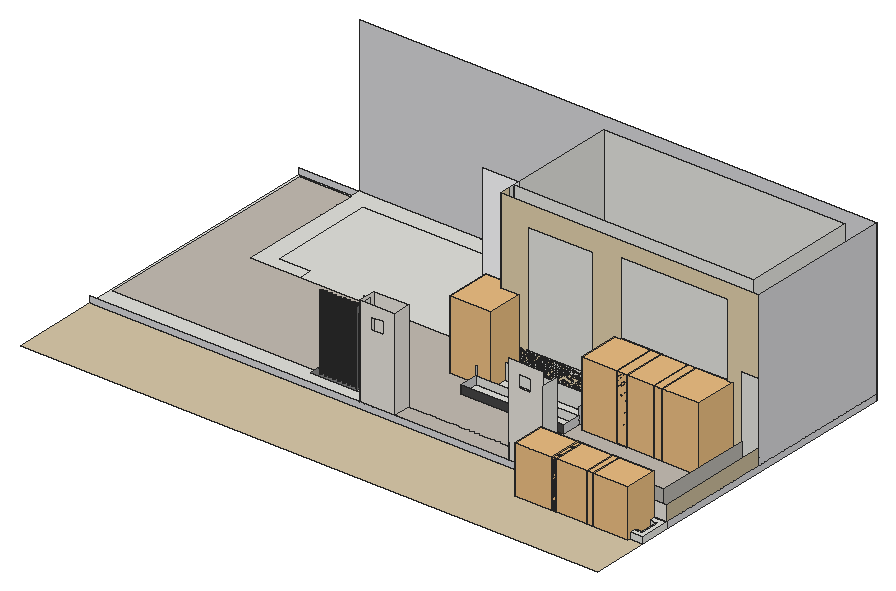
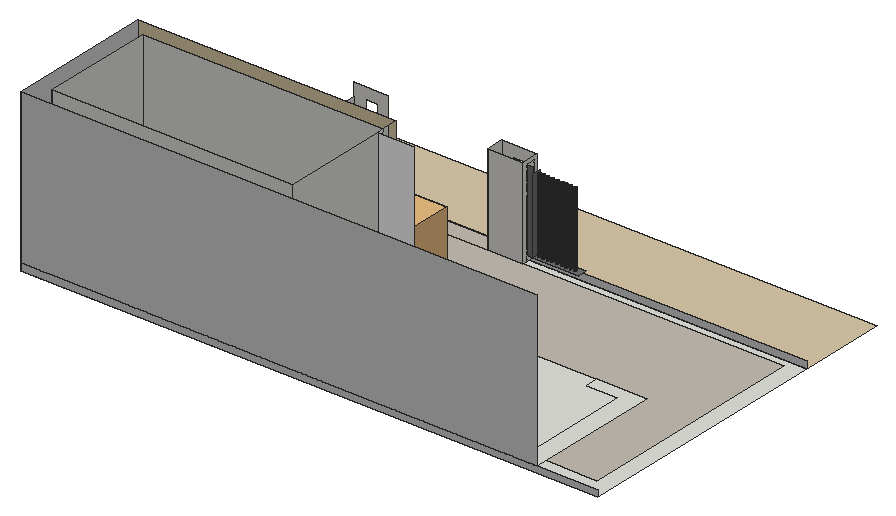
# SketchUp Ruby script. Lengths in inches.
U = 1.inch
M = Sketchup.active_model
def pt(a) = Geom::Point3d.new(a.map { |v| v * U })
def face(e, loops, mat)
  f = e.add_face(loops[0].map { |a| pt(a) })
  loops[1..].each { |l| e.add_face(l.map { |a| pt(a) }).erase! }
  f.material = f.back_material = mat if mat
  f
end
# faces: each face lists its corners as indices into pts; further lists are holes
def faces(e, pts, list, mat = nil) = list.each { |f| face(e, (f[0].is_a?(Array) ? f : [f]).map { |l| l.map { |i| pts[i] } }, mat) }
# xy, xz, yz: faces in a plane at the given z, y or x. An outline is a flat list of corners, or four numbers for a rectangle; further outlines are holes
def ring(l) = l.size == 4 ? [[l[0], l[1]], [l[2], l[1]], [l[2], l[3]], [l[0], l[3]]] : l.each_slice(2).to_a
def flat(e, list, mat, &to3) = list.each { |f| face(e, (f[0].is_a?(Array) ? f : [f]).map { |l| ring(l).map { |u, v| to3.(u, v) } }, mat) }
def xy(e, z, list, mat = nil) = flat(e, list, mat) { |x, y| [x, y, z] }
def xz(e, y, list, mat = nil) = flat(e, list, mat) { |x, z| [x, y, z] }
def yz(e, x, list, mat = nil) = flat(e, list, mat) { |y, z| [x, y, z] }
def lines(e, pts, list) = list.each { |a, b| e.add_line(pt(pts[a]), pt(pts[b])) }
# prism: a flat outline (further loops are holes) pulled along v
def prism(e, loops, v, mat = nil)
  f = face(e, loops, mat); d = Geom::Vector3d.new(v.map { |x| x * U })
  f.pushpull(f.normal.samedirection?(d) ? d.length : -d.length)
end
def box(e, o, s, mat = nil) = prism(e, [[o, [o[0] + s[0], o[1], o[2]], [o[0] + s[0], o[1] + s[1], o[2]], [o[0], o[1] + s[1], o[2]]]], [0, 0, s[2]], mat)
def at(x, y, z, deg = 0) = Geom::Transformation.translation(pt([x, y, z])) * Geom::Transformation.rotation(ORIGIN, Z_AXIS, deg.degrees)
def axes(o, x, y, z) = Geom::Transformation.new([*x, 0, *y, 0, *z, 0, *pt(o).to_a, 1])
def part(name) = M.definitions.add(name)
# library, detail: a bought-in or finely detailed component or shape, given as its bounding box
def library(name, o, s) = part(name).tap { |d| box(d.entities, o, s) }
def detail(e, o, s) = box(e.add_group.entities, o, s)
def put(e, d, t, mat = nil) = e.add_instance(d, t).tap { |i| i.material = mat if mat }
def group(e, t, mat = nil) = e.add_group.tap { |g| g.transformation = t; g.material = mat if mat }.entities
root = M.entities
M.materials.add("[Blinds Vertical Pattern]").color = [212, 212, 214]
M.materials.add("[Carrera Marble]").color = [207, 207, 207]
M.materials.add("[Color M05]").color = [114, 114, 114]
M.materials.add("[Field Rectangle Tile]").color = [196, 189, 179]
M.materials.add("[Field Square Tile]").color = [217, 201, 169]
M.materials.add("[Granite Dark Gray]").color = [69, 68, 68]
M.materials.add("[Quartz Light Brown]").color = [224, 207, 171]
M.materials.add("[Quartz Light Brown]1").color = [199, 184, 152]
M.materials.add("[Quartz Light Grey]").color = [251, 251, 252]
M.materials.add("[Tile Large Brown]").color = [195, 178, 159]
M.materials.add("[Tile Travertine 2 inch]").color = [229, 225, 218]
M.materials.add("[Tile Travertine 2 inch]1").color = [181, 178, 172]
c1 = library("chau cay",[-24.34,-109.24,0],[56.46,62.58,79.69])
c2 = library("Small+Bush+Planter",[-31.86,3.96,0],[62.63,58.8,106.375])
xy(root,0,[[[621.41,77.96,793.87,119.71],[628.97,85.52,786.3125,112.16]],[0,119.71,793.87,479.71]])
xy(root,0,[[0,0,0,119.71,621.41,119.71,621.41,77.96,793.87,77.96,793.87,0]],"[Field Square Tile]")
xy(root,0,[[628.97,85.52,786.3125,112.16]],"[Tile Large Brown]")
xy(root,8.625,[[[621.41,77.96,793.87,119.71],[628.97,85.52,786.3125,112.16]]])
xy(root,9,[[371.37,119.71,419.6875,143.63],[575.77,119.71,622.67,143.63],[622.67,119.71,622.67,143.63,769.95,143.63,769.95,277.72,793.87,277.72,793.87,119.71],[445.64,200.28,587.08,226.75],[445.64,226.75,587.08,253.22],
  [445.64,253.22,587.08,277.72],[769.95,277.72,769.95,455.8,107.23,455.8,107.23,309.84,151.04,309.84,151.04,291.34,83.3125,291.34,83.3125,479.71,793.87,479.71,793.87,277.72],[438.59,277.72,769.95,299.71],[388.47,291.34,438.59,299.71],[438.59,299.71,769.95,455.8]])
xy(root,9,[[419.6875,119.71,575.77,143.63],[12.5625,143.63,769.95,143.63,769.95,277.72,587.08,277.72,587.08,200.28,445.64,200.28,445.64,277.72,438.59,277.72,438.59,291.34,83.3125,291.34,83.3125,464.52,12.5625,464.52]],"[Field Rectangle Tile]")
xy(root,9,[[388.47,299.71,438.59,309.84]],"[Quartz Light Grey]")
xy(root,17.125,[[362.74,125.1875,371.37,137.375],[309.68,129.51,309.27,129.56,308.9,129.72,308.57,129.97,308.32,130.29,308.17,130.67,308.11,131.07,308.17,131.48,308.32,131.86,308.57,132.18,308.9,132.43,309.27,132.58,309.68,132.64,310.08,132.58,310.46,132.43,310.78,132.18,311.03,131.86,311.1875,131.48,311.24,131.07,311.1875,130.67,311.03,130.29,310.78,129.97,310.46,129.72,310.08,129.56],[315.49,129.51,315.09,129.56,314.71,129.72,314.38,129.97,314.14,130.29,313.98,130.67,313.93,131.07,313.98,131.48,314.14,131.86,314.38,132.18,314.71,132.43,315.09,132.58,315.49,132.64,315.89,132.58,316.27,132.43,316.59,132.18,316.84,131.86,317,131.48,317.05,131.07,317,130.67,316.84,130.29,316.59,129.97,316.27,129.72,315.89,129.56],[321.55,129.51,321.15,129.56,320.77,129.72,320.45,129.97,320.2,130.29,320.04,130.67,319.99,131.07,320.04,131.48,320.2,131.86,320.45,132.18,320.77,132.43,321.15,132.58,321.55,132.64,321.96,132.58,322.33,132.43,322.66,132.18,322.91,131.86,323.0625,131.48,323.11,131.07,323.0625,130.67,322.91,130.29,322.66,129.97,322.33,129.72,321.96,129.56],[327.61,129.51,327.21,129.56,326.83,129.72,326.51,129.97,326.26,130.29,326.11,130.67,326.05,131.07,326.11,131.48,326.26,131.86,326.51,132.18,326.83,132.43,327.21,132.58,327.61,132.64,328.02,132.58,328.4,132.43,328.72,132.18,328.97,131.86,329.125,131.48,329.18,131.07,329.125,130.67,328.97,130.29,328.72,129.97,328.4,129.72,328.02,129.56],
  [334.49,129.51,334.09,129.56,333.71,129.72,333.38,129.97,333.14,130.29,332.98,130.67,332.93,131.07,332.98,131.48,333.14,131.86,333.38,132.18,333.71,132.43,334.09,132.58,334.49,132.64,334.89,132.58,335.27,132.43,335.59,132.18,335.84,131.86,336,131.48,336.05,131.07,336,130.67,335.84,130.29,335.59,129.97,335.27,129.72,334.89,129.56],[340.86,129.51,340.46,129.56,340.08,129.72,339.76,129.97,339.51,130.29,339.36,130.67,339.3,131.07,339.36,131.48,339.51,131.86,339.76,132.18,340.08,132.43,340.46,132.58,340.86,132.64,341.27,132.58,341.65,132.43,341.97,132.18,342.22,131.86,342.375,131.48,342.43,131.07,342.375,130.67,342.22,130.29,341.97,129.97,341.65,129.72,341.27,129.56],[347.05,129.51,346.65,129.56,346.27,129.72,345.95,129.97,345.7,130.29,345.54,130.67,345.49,131.07,345.54,131.48,345.7,131.86,345.95,132.18,346.27,132.43,346.65,132.58,347.05,132.64,347.46,132.58,347.83,132.43,348.16,132.18,348.41,131.86,348.5625,131.48,348.61,131.07,348.5625,130.67,348.41,130.29,348.16,129.97,347.83,129.72,347.46,129.56],[353.05,129.51,352.65,129.56,352.27,129.72,351.95,129.97,351.7,130.29,351.54,130.67,351.49,131.07,351.54,131.48,351.7,131.86,351.95,132.18,352.27,132.43,352.65,132.58,353.05,132.64,353.46,132.58,353.83,132.43,354.16,132.18,354.41,131.86,354.5625,131.48,354.61,131.07,354.5625,130.67,354.41,130.29,354.16,129.97,353.83,129.72,353.46,129.56],[358.68,129.51,358.27,129.56,357.9,129.72,357.57,129.97,357.32,130.29,357.17,130.67,357.11,131.07,357.17,131.48,357.32,131.86,357.57,132.18,357.9,132.43,358.27,132.58,358.68,132.64,359.08,132.58,359.46,132.43,359.78,132.18,360.03,131.86,360.1875,131.48,360.24,131.07,360.1875,130.67,360.03,130.29,359.78,129.97,359.46,129.72,359.08,129.56]])
xy(root,17.125,[[[299.8,125.1875,362.74,137.375],[303.86,129.51,303.46,129.56,303.08,129.72,302.76,129.97,302.51,130.29,302.36,130.67,302.3,131.07,302.36,131.48,302.51,131.86,302.76,132.18,303.08,132.43,303.46,132.58,303.86,132.64,304.27,132.58,304.65,132.43,304.97,132.18,305.22,131.86,305.375,131.48,305.43,131.07,305.375,130.67,305.22,130.29,304.97,129.97,304.65,129.72,304.27,129.56],[358.68,129.51,358.27,129.56,357.9,129.72,357.57,129.97,357.32,130.29,357.17,130.67,357.11,131.07,357.17,131.48,357.32,131.86,357.57,132.18,357.9,132.43,358.27,132.58,358.68,132.64,359.08,132.58,359.46,132.43,359.78,132.18,360.03,131.86,360.1875,131.48,360.24,131.07,360.1875,130.67,360.03,130.29,359.78,129.97,359.46,129.72,359.08,129.56],[309.68,129.51,309.27,129.56,308.9,129.72,308.57,129.97,308.32,130.29,308.17,130.67,308.11,131.07,308.17,131.48,308.32,131.86,308.57,132.18,308.9,132.43,309.27,132.58,309.68,132.64,310.08,132.58,310.46,132.43,310.78,132.18,311.03,131.86,311.1875,131.48,311.24,131.07,311.1875,130.67,311.03,130.29,310.78,129.97,310.46,129.72,310.08,129.56],[353.05,129.51,352.65,129.56,352.27,129.72,351.95,129.97,351.7,130.29,351.54,130.67,351.49,131.07,351.54,131.48,351.7,131.86,351.95,132.18,352.27,132.43,352.65,132.58,353.05,132.64,353.46,132.58,353.83,132.43,354.16,132.18,354.41,131.86,354.5625,131.48,354.61,131.07,354.5625,130.67,354.41,130.29,354.16,129.97,353.83,129.72,353.46,129.56],[315.49,129.51,315.09,129.56,314.71,129.72,314.38,129.97,314.14,130.29,313.98,130.67,313.93,131.07,313.98,131.48,314.14,131.86,314.38,132.18,314.71,132.43,315.09,132.58,315.49,132.64,315.89,132.58,316.27,132.43,316.59,132.18,316.84,131.86,317,131.48,317.05,131.07,317,130.67,316.84,130.29,316.59,129.97,316.27,129.72,315.89,129.56],[347.05,129.51,346.65,129.56,346.27,129.72,345.95,129.97,345.7,130.29,345.54,130.67,345.49,131.07,345.54,131.48,345.7,131.86,345.95,132.18,346.27,132.43,346.65,132.58,347.05,132.64,347.46,132.58,347.83,132.43,348.16,132.18,348.41,131.86,348.5625,131.48,348.61,131.07,348.5625,130.67,348.41,130.29,348.16,129.97,347.83,129.72,347.46,129.56],[321.55,129.51,321.15,129.56,320.77,129.72,320.45,129.97,320.2,130.29,320.04,130.67,319.99,131.07,320.04,131.48,320.2,131.86,320.45,132.18,320.77,132.43,321.15,132.58,321.55,132.64,321.96,132.58,322.33,132.43,322.66,132.18,322.91,131.86,323.0625,131.48,323.11,131.07,323.0625,130.67,322.91,130.29,322.66,129.97,322.33,129.72,321.96,129.56],[340.86,129.51,340.46,129.56,340.08,129.72,339.76,129.97,339.51,130.29,339.36,130.67,339.3,131.07,339.36,131.48,339.51,131.86,339.76,132.18,340.08,132.43,340.46,132.58,340.86,132.64,341.27,132.58,341.65,132.43,341.97,132.18,342.22,131.86,342.375,131.48,342.43,131.07,342.375,130.67,342.22,130.29,341.97,129.97,341.65,129.72,341.27,129.56],[327.61,129.51,327.21,129.56,326.83,129.72,326.51,129.97,326.26,130.29,326.11,130.67,326.05,131.07,326.11,131.48,326.26,131.86,326.51,132.18,326.83,132.43,327.21,132.58,327.61,132.64,328.02,132.58,328.4,132.43,328.72,132.18,328.97,131.86,329.125,131.48,329.18,131.07,329.125,130.67,328.97,130.29,328.72,129.97,328.4,129.72,328.02,129.56],[334.49,129.51,334.09,129.56,333.71,129.72,333.38,129.97,333.14,130.29,332.98,130.67,332.93,131.07,332.98,131.48,333.14,131.86,333.38,132.18,333.71,132.43,334.09,132.58,334.49,132.64,334.89,132.58,335.27,132.43,335.59,132.18,335.84,131.86,336,131.48,336.05,131.07,336,130.67,335.84,130.29,335.59,129.97,335.27,129.72,334.89,129.56]]],"[Color M05]")
xz(root,77.96,[[621.41,0,793.87,8.625]])
xz(root,85.52,[[628.97,0,786.3125,8.625]])
xz(root,112.16,[[628.97,0,786.3125,8.625]])
xz(root,119.71,[[621.41,0,793.87,8.625]])
xz(root,119.71,[[0,0,621.41,0,621.41,8.625,793.87,8.625,793.87,9,0,9]],"[Blinds Vertical Pattern]")
xz(root,119.71,[[[371.37,9,419.6875,133.9375],[387.01,102.5625,403.76,119.3125]],[[575.77,9,622.67,133.9375],[590.2,102.5625,606.95,119.3125]],[622.67,9,793.87,30.25]],"[Tile Travertine 2 inch]")
xz(root,137.375,[[362.74,17.125,371.37,128.625]],"[Color M05]")
xz(root,143.63,[[371.37,9,419.6875,133.9375],[575.77,9,622.67,30.25]],"[Tile Travertine 2 inch]")
xz(root,143.63,[[622.67,9,769.95,30.25]],"[Tile Travertine 2 inch]1")
xz(root,200.28,[[445.64,9,587.08,20.25]],"[Granite Dark Gray]")
xz(root,226.75,[[445.64,9,587.08,20.25]])
xz(root,253.22,[[445.64,9,587.08,31.375]])
xz(root,277.72,[[445.64,9,587.08,39.19],[769.95,9,793.87,116.1875]])
xz(root,277.72,[[[438.59,9,769.95,9,769.95,116.1875,793.87,116.1875,793.87,220,438.59,220],[604.02,43.13,751.39,199.88],[476.45,39.19,566.07,192.07]]],"[Quartz Light Brown]")
xz(root,299.71,[[438.59,9,769.95,220]])
xz(root,309.84,[[388.47,9,438.59,220]],"[Quartz Light Grey]")
xz(root,455.8,[[438.59,9,769.95,220]])
xz(root,479.71,[[0,0,793.87,9],[83.3125,9,793.87,220]],"[Blinds Vertical Pattern]")
yz(root,362.74,[[125.1875,17.125,137.375,119.59]],"[Color M05]")
yz(root,371.37,[[125.1875,9,137.375,17.125],[125.1875,17.125,137.375,128.625]])
yz(root,371.37,[[119.71,9,119.71,133.9375,143.63,133.9375,143.63,9,137.375,9,137.375,128.625,125.1875,128.625,125.1875,9]],"[Tile Travertine 2 inch]")
yz(root,388.47,[[299.71,9,309.84,38.0625]])
yz(root,419.6875,[[119.71,9,143.63,133.9375]],"[Tile Travertine 2 inch]")
yz(root,438.59,[[291.34,9,299.71,220],[309.84,9,455.8,220]])
yz(root,438.59,[[277.72,9,291.34,220]],"[Quartz Light Brown]")
yz(root,438.59,[[299.71,9,309.84,220]],"[Quartz Light Grey]")
yz(root,445.64,[[200.28,9,226.75,20.25],[226.75,9,253.22,31.375],[253.22,9,277.72,39.19]],"[Carrera Marble]")
yz(root,575.77,[[119.71,9,143.63,30.25]],"[Tile Travertine 2 inch]")
yz(root,587.08,[[200.28,9,226.75,20.25],[226.75,9,253.22,31.375],[253.22,9,277.72,39.19]],"[Carrera Marble]")
yz(root,621.41,[[77.96,0,119.71,8.625]])
yz(root,622.67,[[119.71,9,143.63,116.1875]])
yz(root,628.97,[[85.52,0,112.16,8.625]])
yz(root,769.95,[[299.71,9,455.8,220]])
yz(root,769.95,[[143.63,9,277.72,30.25]],"[Tile Travertine 2 inch]1")
yz(root,786.3125,[[85.52,0,112.16,8.625]])
yz(root,793.87,[[77.96,0,119.71,8.625]])
yz(root,793.87,[[119.71,0,479.71,9],[277.72,9,479.71,220]],"[Blinds Vertical Pattern]")
yz(root,793.87,[[119.71,9,277.72,30.25]],"[Quartz Light Brown]1")
p = [[309.27,129.56,17.125],[309.68,129.51,17.125],[309.68,129.51,119.59],[309.27,129.56,119.59],[310.08,129.56,17.125],[310.08,129.56,119.59],
  [315.09,129.56,17.125],[315.49,129.51,17.125],[315.49,129.51,119.59],[315.09,129.56,119.59],[315.89,129.56,17.125],[315.89,129.56,119.59],
  [321.15,129.56,17.125],[321.55,129.51,17.125],[321.55,129.51,119.59],[321.15,129.56,119.59],[321.96,129.56,17.125],[321.96,129.56,119.59],
  [327.21,129.56,17.125],[327.61,129.51,17.125],[327.61,129.51,119.59],[327.21,129.56,119.59],[328.02,129.56,17.125],[328.02,129.56,119.59],
  [334.09,129.56,17.125],[334.49,129.51,17.125],[334.49,129.51,119.59],[334.09,129.56,119.59],[334.89,129.56,17.125],[334.89,129.56,119.59],
  [340.46,129.56,17.125],[340.86,129.51,17.125],[340.86,129.51,119.59],[340.46,129.56,119.59],[341.27,129.56,17.125],[341.27,129.56,119.59],
  [346.65,129.56,17.125],[347.05,129.51,17.125],[347.05,129.51,119.59],[346.65,129.56,119.59],[347.46,129.56,17.125],[347.46,129.56,119.59],
  [352.65,129.56,17.125],[353.05,129.51,17.125],[353.05,129.51,119.59],[352.65,129.56,119.59],[353.46,129.56,17.125],[353.46,129.56,119.59],
  [358.27,129.56,17.125],[358.68,129.51,17.125],[358.68,129.51,119.59],[358.27,129.56,119.59],[359.08,129.56,17.125],[359.08,129.56,119.59],
  [308.9,129.72,17.125],[308.9,129.72,119.59],[310.46,129.72,17.125],[310.46,129.72,119.59],[314.71,129.72,17.125],[314.71,129.72,119.59],
  [316.27,129.72,17.125],[316.27,129.72,119.59],[320.77,129.72,17.125],[320.77,129.72,119.59],[322.33,129.72,17.125],[322.33,129.72,119.59],
  [326.83,129.72,17.125],[326.83,129.72,119.59],[328.4,129.72,17.125],[328.4,129.72,119.59],[333.71,129.72,17.125],[333.71,129.72,119.59],
  [335.27,129.72,17.125],[335.27,129.72,119.59],[340.08,129.72,17.125],[340.08,129.72,119.59],[341.65,129.72,17.125],[341.65,129.72,119.59],
  [346.27,129.72,17.125],[346.27,129.72,119.59],[347.83,129.72,17.125],[347.83,129.72,119.59],[352.27,129.72,17.125],[352.27,129.72,119.59],
  [353.83,129.72,17.125],[353.83,129.72,119.59],[357.9,129.72,17.125],[357.9,129.72,119.59],[359.46,129.72,17.125],[359.46,129.72,119.59],
  [308.57,129.97,17.125],[308.57,129.97,119.59],[310.78,129.97,17.125],[310.78,129.97,119.59],[314.38,129.97,17.125],[314.38,129.97,119.59],
  [316.59,129.97,17.125],[316.59,129.97,119.59],[320.45,129.97,17.125],[320.45,129.97,119.59],[322.66,129.97,17.125],[322.66,129.97,119.59],
  [326.51,129.97,17.125],[326.51,129.97,119.59],[328.72,129.97,17.125],[328.72,129.97,119.59],[333.38,129.97,17.125],[333.38,129.97,119.59],
  [335.59,129.97,17.125],[335.59,129.97,119.59],[339.76,129.97,17.125],[339.76,129.97,119.59],[341.97,129.97,17.125],[341.97,129.97,119.59],
  [345.95,129.97,17.125],[345.95,129.97,119.59],[348.16,129.97,17.125],[348.16,129.97,119.59],[351.95,129.97,17.125],[351.95,129.97,119.59],
  [354.16,129.97,17.125],[354.16,129.97,119.59],[357.57,129.97,17.125],[357.57,129.97,119.59],[359.78,129.97,17.125],[359.78,129.97,119.59],
  [308.32,130.29,17.125],[308.32,130.29,119.59],[311.03,130.29,17.125],[311.03,130.29,119.59],[314.14,130.29,17.125],[314.14,130.29,119.59],
  [316.84,130.29,17.125],[316.84,130.29,119.59],[320.2,130.29,17.125],[320.2,130.29,119.59],[322.91,130.29,17.125],[322.91,130.29,119.59],
  [326.26,130.29,17.125],[326.26,130.29,119.59],[328.97,130.29,17.125],[328.97,130.29,119.59],[333.14,130.29,17.125],[333.14,130.29,119.59],
  [335.84,130.29,17.125],[335.84,130.29,119.59],[339.51,130.29,17.125],[339.51,130.29,119.59],[342.22,130.29,17.125],[342.22,130.29,119.59],
  [345.7,130.29,17.125],[345.7,130.29,119.59],[348.41,130.29,17.125],[348.41,130.29,119.59],[351.7,130.29,17.125],[351.7,130.29,119.59],
  [354.41,130.29,17.125],[354.41,130.29,119.59],[357.32,130.29,17.125],[357.32,130.29,119.59],[360.03,130.29,17.125],[360.03,130.29,119.59],
  [308.17,130.67,17.125],[308.17,130.67,119.59],[311.1875,130.67,17.125],[311.1875,130.67,119.59],[313.98,130.67,17.125],[313.98,130.67,119.59],
  [317,130.67,17.125],[317,130.67,119.59],[320.04,130.67,17.125],[320.04,130.67,119.59],[323.0625,130.67,17.125],[323.0625,130.67,119.59],
  [326.11,130.67,17.125],[326.11,130.67,119.59],[329.125,130.67,17.125],[329.125,130.67,119.59],[332.98,130.67,17.125],[332.98,130.67,119.59],
  [336,130.67,17.125],[336,130.67,119.59],[339.36,130.67,17.125],[339.36,130.67,119.59],[342.375,130.67,17.125],[342.375,130.67,119.59],
  [345.54,130.67,17.125],[345.54,130.67,119.59],[348.5625,130.67,17.125],[348.5625,130.67,119.59],[351.54,130.67,17.125],[351.54,130.67,119.59],
  [354.5625,130.67,17.125],[354.5625,130.67,119.59],[357.17,130.67,17.125],[357.17,130.67,119.59],[360.1875,130.67,17.125],[360.1875,130.67,119.59],
  [308.11,131.07,17.125],[308.11,131.07,119.59],[311.24,131.07,17.125],[311.24,131.07,119.59],[313.93,131.07,17.125],[313.93,131.07,119.59],
  [317.05,131.07,17.125],[317.05,131.07,119.59],[319.99,131.07,17.125],[319.99,131.07,119.59],[323.11,131.07,17.125],[323.11,131.07,119.59],
  [326.05,131.07,17.125],[326.05,131.07,119.59],[329.18,131.07,17.125],[329.18,131.07,119.59],[332.93,131.07,17.125],[332.93,131.07,119.59],
  [336.05,131.07,17.125],[336.05,131.07,119.59],[339.3,131.07,17.125],[339.3,131.07,119.59],[342.43,131.07,17.125],[342.43,131.07,119.59],
  [345.49,131.07,17.125],[345.49,131.07,119.59],[348.61,131.07,17.125],[348.61,131.07,119.59],[351.49,131.07,17.125],[351.49,131.07,119.59],
  [354.61,131.07,17.125],[354.61,131.07,119.59],[357.11,131.07,17.125],[357.11,131.07,119.59],[360.24,131.07,17.125],[360.24,131.07,119.59],
  [311.1875,131.48,17.125],[311.1875,131.48,119.59],[313.98,131.48,17.125],[313.98,131.48,119.59],[317,131.48,17.125],[317,131.48,119.59],
  [320.04,131.48,17.125],[320.04,131.48,119.59],[323.0625,131.48,17.125],[323.0625,131.48,119.59],[326.11,131.48,17.125],[326.11,131.48,119.59],
  [329.125,131.48,17.125],[329.125,131.48,119.59],[332.98,131.48,17.125],[332.98,131.48,119.59],[336,131.48,17.125],[336,131.48,119.59],
  [339.36,131.48,17.125],[339.36,131.48,119.59],[342.375,131.48,17.125],[342.375,131.48,119.59],[345.54,131.48,17.125],[345.54,131.48,119.59],
  [348.5625,131.48,17.125],[348.5625,131.48,119.59],[351.54,131.48,17.125],[351.54,131.48,119.59],[354.5625,131.48,17.125],[354.5625,131.48,119.59],
  [357.17,131.48,17.125],[357.17,131.48,119.59],[360.1875,131.48,17.125],[360.1875,131.48,119.59],[308.32,131.86,17.125],[308.17,131.48,17.125],
  [308.17,131.48,119.59],[308.32,131.86,119.59],[311.03,131.86,17.125],[311.03,131.86,119.59],[314.14,131.86,17.125],[314.14,131.86,119.59],
  [316.84,131.86,17.125],[316.84,131.86,119.59],[320.2,131.86,17.125],[320.2,131.86,119.59],[322.91,131.86,17.125],[322.91,131.86,119.59],
  [326.26,131.86,17.125],[326.26,131.86,119.59],[328.97,131.86,17.125],[328.97,131.86,119.59],[333.14,131.86,17.125],[333.14,131.86,119.59],
  [335.84,131.86,17.125],[335.84,131.86,119.59],[339.51,131.86,17.125],[339.51,131.86,119.59],[342.22,131.86,17.125],[342.22,131.86,119.59],
  [345.7,131.86,17.125],[345.7,131.86,119.59],[348.41,131.86,17.125],[348.41,131.86,119.59],[351.7,131.86,17.125],[351.7,131.86,119.59],
  [354.41,131.86,17.125],[354.41,131.86,119.59],[357.32,131.86,17.125],[357.32,131.86,119.59],[360.03,131.86,17.125],[360.03,131.86,119.59],
  [308.57,132.18,17.125],[308.57,132.18,119.59],[310.78,132.18,17.125],[310.78,132.18,119.59],[314.38,132.18,17.125],[314.38,132.18,119.59],
  [316.59,132.18,17.125],[316.59,132.18,119.59],[320.45,132.18,17.125],[320.45,132.18,119.59],[322.66,132.18,17.125],[322.66,132.18,119.59],
  [326.51,132.18,17.125],[326.51,132.18,119.59],[328.72,132.18,17.125],[328.72,132.18,119.59],[333.38,132.18,17.125],[333.38,132.18,119.59],
  [335.59,132.18,17.125],[335.59,132.18,119.59],[339.76,132.18,17.125],[339.76,132.18,119.59],[341.97,132.18,17.125],[341.97,132.18,119.59],
  [345.95,132.18,17.125],[345.95,132.18,119.59],[348.16,132.18,17.125],[348.16,132.18,119.59],[351.95,132.18,17.125],[351.95,132.18,119.59],
  [354.16,132.18,17.125],[354.16,132.18,119.59],[357.57,132.18,17.125],[357.57,132.18,119.59],[359.78,132.18,17.125],[359.78,132.18,119.59],
  [308.9,132.43,17.125],[308.9,132.43,119.59],[310.46,132.43,17.125],[310.46,132.43,119.59],[314.71,132.43,17.125],[314.71,132.43,119.59],
  [316.27,132.43,17.125],[316.27,132.43,119.59],[320.77,132.43,17.125],[320.77,132.43,119.59],[322.33,132.43,17.125],[322.33,132.43,119.59],
  [326.83,132.43,17.125],[326.83,132.43,119.59],[328.4,132.43,17.125],[328.4,132.43,119.59],[333.71,132.43,17.125],[333.71,132.43,119.59],
  [335.27,132.43,17.125],[335.27,132.43,119.59],[340.08,132.43,17.125],[340.08,132.43,119.59],[341.65,132.43,17.125],[341.65,132.43,119.59],
  [346.27,132.43,17.125],[346.27,132.43,119.59],[347.83,132.43,17.125],[347.83,132.43,119.59],[352.27,132.43,17.125],[352.27,132.43,119.59],
  [353.83,132.43,17.125],[353.83,132.43,119.59],[357.9,132.43,17.125],[357.9,132.43,119.59],[359.46,132.43,17.125],[359.46,132.43,119.59],
  [309.27,132.58,17.125],[309.27,132.58,119.59],[310.08,132.58,17.125],[310.08,132.58,119.59],[315.09,132.58,17.125],[315.09,132.58,119.59],
  [315.89,132.58,17.125],[315.89,132.58,119.59],[321.15,132.58,17.125],[321.15,132.58,119.59],[321.96,132.58,17.125],[321.96,132.58,119.59],
  [327.21,132.58,17.125],[327.21,132.58,119.59],[328.02,132.58,17.125],[328.02,132.58,119.59],[334.09,132.58,17.125],[334.09,132.58,119.59],
  [334.89,132.58,17.125],[334.89,132.58,119.59],[340.46,132.58,17.125],[340.46,132.58,119.59],[341.27,132.58,17.125],[341.27,132.58,119.59],
  [346.65,132.58,17.125],[346.65,132.58,119.59],[347.46,132.58,17.125],[347.46,132.58,119.59],[352.65,132.58,17.125],[352.65,132.58,119.59],
  [353.46,132.58,17.125],[353.46,132.58,119.59],[358.27,132.58,17.125],[358.27,132.58,119.59],[359.08,132.58,17.125],[359.08,132.58,119.59],
  [309.68,132.64,17.125],[309.68,132.64,119.59],[315.49,132.64,17.125],[315.49,132.64,119.59],[321.55,132.64,17.125],[321.55,132.64,119.59],
  [327.61,132.64,17.125],[327.61,132.64,119.59],[334.49,132.64,17.125],[334.49,132.64,119.59],[340.86,132.64,17.125],[340.86,132.64,119.59],
  [347.05,132.64,17.125],[347.05,132.64,119.59],[353.05,132.64,17.125],[353.05,132.64,119.59],[358.68,132.64,17.125],[358.68,132.64,119.59]]
faces(root,p,[[0,1,2,3],[1,4,5,2],[6,7,8,9],[7,10,11,8],[12,13,14,15],[13,16,17,14],[18,19,20,21],[19,22,23,20],
  [24,25,26,27],[25,28,29,26],[30,31,32,33],[31,34,35,32],[36,37,38,39],[37,40,41,38],[42,43,44,45],[43,46,47,44],
  [48,49,50,51],[49,52,53,50],[54,0,3,55],[4,56,57,5],[58,6,9,59],[10,60,61,11],[62,12,15,63],[16,64,65,17],
  [66,18,21,67],[22,68,69,23],[70,24,27,71],[28,72,73,29],[74,30,33,75],[34,76,77,35],[78,36,39,79],[40,80,81,41],
  [82,42,45,83],[46,84,85,47],[86,48,51,87],[52,88,89,53],[90,54,55,91],[56,92,93,57],[94,58,59,95],[60,96,97,61],
  [98,62,63,99],[64,100,101,65],[102,66,67,103],[68,104,105,69],[106,70,71,107],[72,108,109,73],[110,74,75,111],[76,112,113,77],
  [114,78,79,115],[80,116,117,81],[118,82,83,119],[84,120,121,85],[122,86,87,123],[88,124,125,89],[126,90,91,127],[92,128,129,93],
  [130,94,95,131],[96,132,133,97],[134,98,99,135],[100,136,137,101],[138,102,103,139],[104,140,141,105],[142,106,107,143],[108,144,145,109],
  [146,110,111,147],[112,148,149,113],[150,114,115,151],[116,152,153,117],[154,118,119,155],[120,156,157,121],[158,122,123,159],[124,160,161,125],
  [162,126,127,163],[128,164,165,129],[166,130,131,167],[132,168,169,133],[170,134,135,171],[136,172,173,137],[174,138,139,175],[140,176,177,141],
  [178,142,143,179],[144,180,181,145],[182,146,147,183],[148,184,185,149],[186,150,151,187],[152,188,189,153],[190,154,155,191],[156,192,193,157],
  [194,158,159,195],[160,196,197,161],[198,162,163,199],[164,200,201,165],[202,166,167,203],[168,204,205,169],[206,170,171,207],[172,208,209,173],
  [210,174,175,211],[176,212,213,177],[214,178,179,215],[180,216,217,181],[218,182,183,219],[184,220,221,185],[222,186,187,223],[188,224,225,189],
  [226,190,191,227],[192,228,229,193],[230,194,195,231],[196,232,233,197],[200,234,235,201],[236,202,203,237],[204,238,239,205],[240,206,207,241],
  [208,242,243,209],[244,210,211,245],[212,246,247,213],[248,214,215,249],[216,250,251,217],[252,218,219,253],[220,254,255,221],[256,222,223,257],
  [224,258,259,225],[260,226,227,261],[228,262,263,229],[264,230,231,265],[232,266,267,233],[268,269,270,271],[234,272,273,235],[274,236,237,275],
  [238,276,277,239],[278,240,241,279],[242,280,281,243],[282,244,245,283],[246,284,285,247],[286,248,249,287],[250,288,289,251],[290,252,253,291],
  [254,292,293,255],[294,256,257,295],[258,296,297,259],[298,260,261,299],[262,300,301,263],[302,264,265,303],[266,304,305,267],[306,268,271,307],
  [272,308,309,273],[310,274,275,311],[276,312,313,277],[314,278,279,315],[280,316,317,281],[318,282,283,319],[284,320,321,285],[322,286,287,323],
  [288,324,325,289],[326,290,291,327],[292,328,329,293],[330,294,295,331],[296,332,333,297],[334,298,299,335],[300,336,337,301],[338,302,303,339],
  [304,340,341,305],[342,306,307,343],[308,344,345,309],[346,310,311,347],[312,348,349,313],[350,314,315,351],[316,352,353,317],[354,318,319,355],
  [320,356,357,321],[358,322,323,359],[324,360,361,325],[362,326,327,363],[328,364,365,329],[366,330,331,367],[332,368,369,333],[370,334,335,371],
  [336,372,373,337],[374,338,339,375],[340,376,377,341],[378,342,343,379],[344,380,381,345],[382,346,347,383],[348,384,385,349],[386,350,351,387],
  [352,388,389,353],[390,354,355,391],[356,392,393,357],[394,358,359,395],[360,396,397,361],[398,362,363,399],[364,400,401,365],[402,366,367,403],
  [368,404,405,369],[406,370,371,407],[372,408,409,373],[410,374,375,411],[376,412,413,377],[414,378,379,415],[380,414,415,381],[416,382,383,417],
  [384,416,417,385],[418,386,387,419],[388,418,419,389],[420,390,391,421],[392,420,421,393],[422,394,395,423],[396,422,423,397],[424,398,399,425],
  [400,424,425,401],[426,402,403,427],[404,426,427,405],[428,406,407,429],[408,428,429,409],[430,410,411,431],[412,430,431,413]],"[Color M05]")
put(root,c1,axes([431.74,338,9],[1,0,0],[0,1,0],[0,0,1.19]))
put(root,c2,axes([627.76,216.4,9],[1,0,0],[0,1,0],[0,0,0.84]))
put(root,c2,axes([649.3125,72.02,0],[0.9,0,0],[0,0.76,0],[0,0,0.61354]))
put(root,c2,axes([675.82,216.4,9],[1,0,0],[0,1,0],[0,0,0.84]))
put(root,c2,axes([700.1875,72.02,0],[0.9,0,0],[0,0.76,0],[0,0,0.61354]))
put(root,c2,axes([727.07,216.4,9],[1,0,0],[0,1,0],[0,0,0.84]))
put(root,c2,axes([748.125,72.02,0],[0.9,0,0],[0,0.76,0],[0,0,0.61354]))
